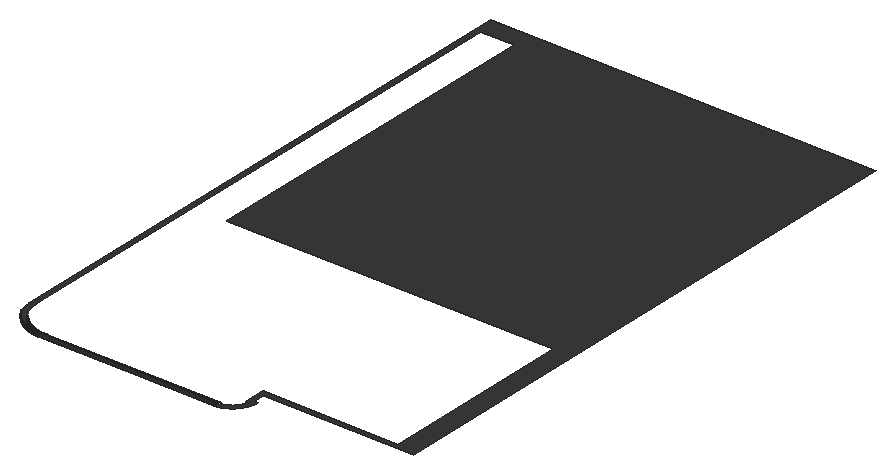
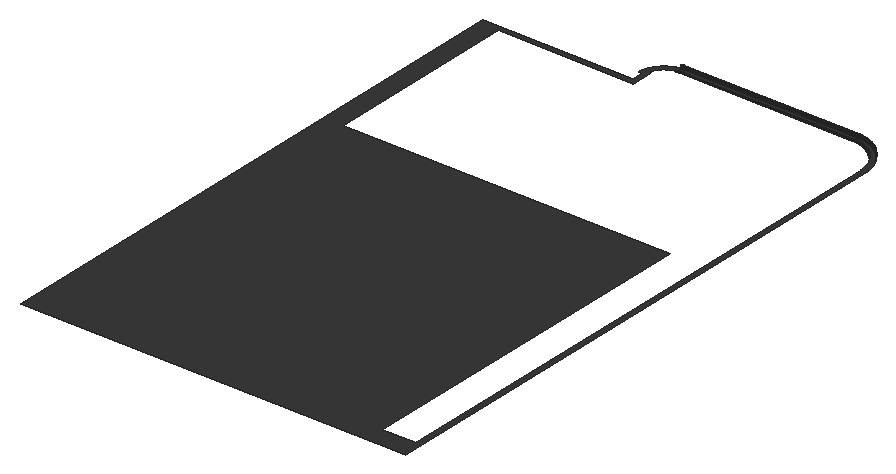
# SketchUp Ruby script. Lengths in inches.
U = 1.inch
M = Sketchup.active_model
def pt(a) = Geom::Point3d.new(a.map { |v| v * U })
def face(e, loops, mat)
  f = e.add_face(loops[0].map { |a| pt(a) })
  loops[1..].each { |l| e.add_face(l.map { |a| pt(a) }).erase! }
  f.material = f.back_material = mat if mat
  f
end
# faces: each face lists its corners as indices into pts; further lists are holes
def faces(e, pts, list, mat = nil) = list.each { |f| face(e, (f[0].is_a?(Array) ? f : [f]).map { |l| l.map { |i| pts[i] } }, mat) }
# xy, xz, yz: faces in a plane at the given z, y or x. An outline is a flat list of corners, or four numbers for a rectangle; further outlines are holes
def ring(l) = l.size == 4 ? [[l[0], l[1]], [l[2], l[1]], [l[2], l[3]], [l[0], l[3]]] : l.each_slice(2).to_a
def flat(e, list, mat, &to3) = list.each { |f| face(e, (f[0].is_a?(Array) ? f : [f]).map { |l| ring(l).map { |u, v| to3.(u, v) } }, mat) }
def xy(e, z, list, mat = nil) = flat(e, list, mat) { |x, y| [x, y, z] }
def xz(e, y, list, mat = nil) = flat(e, list, mat) { |x, z| [x, y, z] }
def yz(e, x, list, mat = nil) = flat(e, list, mat) { |y, z| [x, y, z] }
def lines(e, pts, list) = list.each { |a, b| e.add_line(pt(pts[a]), pt(pts[b])) }
# prism: a flat outline (further loops are holes) pulled along v
def prism(e, loops, v, mat = nil)
  f = face(e, loops, mat); d = Geom::Vector3d.new(v.map { |x| x * U })
  f.pushpull(f.normal.samedirection?(d) ? d.length : -d.length)
end
def box(e, o, s, mat = nil) = prism(e, [[o, [o[0] + s[0], o[1], o[2]], [o[0] + s[0], o[1] + s[1], o[2]], [o[0], o[1] + s[1], o[2]]]], [0, 0, s[2]], mat)
def at(x, y, z, deg = 0) = Geom::Transformation.translation(pt([x, y, z])) * Geom::Transformation.rotation(ORIGIN, Z_AXIS, deg.degrees)
def axes(o, x, y, z) = Geom::Transformation.new([*x, 0, *y, 0, *z, 0, *pt(o).to_a, 1])
def part(name) = M.definitions.add(name)
# library, detail: a bought-in or finely detailed component or shape, given as its bounding box
def library(name, o, s) = part(name).tap { |d| box(d.entities, o, s) }
def detail(e, o, s) = box(e.add_group.entities, o, s)
def put(e, d, t, mat = nil) = e.add_instance(d, t).tap { |i| i.material = mat if mat }
def group(e, t, mat = nil) = e.add_group.tap { |g| g.transformation = t; g.material = mat if mat }.entities
root = M.entities
M.materials.add("1496 AP 8293 CARBON COPY").color = [58, 58, 58]
xy(root,258,[[[43.57,64,43.14,64.01,42.7,64.03,41.84,64.07,41.41,64.1,40.55,64.18,39.69,64.28,39.26,64.34,38.84,64.41,38.41,64.48,37.99,64.55,37.5625,64.63,37.14,64.72,36.72,64.8125,36.3,64.91,35.875,65.02,35.46,65.125,35.04,65.24,34.63,65.36,34.21,65.48,33.8,65.62,33.39,65.75,32.98,65.89,32.58,66.04,32.17,66.19,31.37,66.51,30.97,66.68,30.58,66.85,30.18,67.03,29.79,67.21,29.4,67.4,29.02,67.6,28.63,67.8,28.25,68,27.5,68.42,26.76,68.86,26.39,69.09,26.03,69.32,25.67,69.5625,25.31,69.8,24.95,70.05,24.6,70.3,24.26,70.56,23.91,70.82,23.57,71.08,23.23,71.35,22.57,71.91,22.24,72.1875,21.92,72.48,21.6,72.77,21.28,73.0625,20.97,73.36,20.67,73.67,20.36,73.97,20.0625,74.28,19.77,74.6,19.48,74.92,19.1875,75.24,18.91,75.57,18.35,76.23,18.08,76.57,17.82,76.91,17.56,77.26,17.3,77.6,17.05,77.95,16.8,78.31,16.5625,78.67,16.32,79.03,16.09,79.39,15.86,79.76,15.42,80.5,15,81.25,14.8,81.63,14.6,82.02,14.4,82.4,14.21,82.79,14.03,83.18,13.85,83.58,13.68,83.97,13.51,84.37,13.19,85.17,13.04,85.58,12.89,85.98,12.75,86.39,12.62,86.8,12.48,87.21,12.36,87.63,12.24,88.04,12.125,88.46,12.02,88.875,11.91,89.3,11.8125,89.72,11.72,90.14,11.63,90.5625,11.55,90.99,11.48,91.41,11.41,91.84,11.34,92.26,11.28,92.69,11.18,93.55,11.1,94.41,11.07,94.84,11.03,95.7,11.01,96.14,11,96.57,11,567,326,567,326,94,203,94,203,85,206,85,206,84.73,205.99,84.45,205.98,84.18,205.97,83.9,205.96,83.625,205.94,83.35,205.91,83.08,205.88,82.8,205.82,82.26,205.78,81.99,205.74,81.71,205.7,81.44,205.6,80.9,205.54,80.63,205.48,80.37,205.42,80.1,205.28,79.56,205.14,79.04,205.06,78.77,204.97,78.51,204.89,78.25,204.8,77.99,204.7,77.73,204.61,77.47,204.51,77.22,204.4,76.96,204.07,76.21,203.83,75.71,203.71,75.47,203.58,75.22,203.46,74.98,203.32,74.74,203.1875,74.5,203.05,74.26,202.91,74.03,202.76,73.79,202.61,73.5625,202.46,73.33,202.31,73.11,202.15,72.88,201.83,72.44,201.32,71.78,201.15,71.57,200.79,71.15,200.61,70.95,200.42,70.75,200.23,70.54,200.04,70.35,199.85,70.15,199.65,69.96,199.46,69.77,199.25,69.58,199.05,69.39,198.85,69.21,198.43,68.85,198.22,68.68,197.56,68.17,197.12,67.85,196.89,67.69,196.67,67.54,196.4375,67.39,196.21,67.24,195.97,67.09,195.74,66.95,195.5,66.8125,195.26,66.68,195.02,66.54,194.78,66.42,194.53,66.29,194.29,66.17,193.79,65.93,193.04,65.6,192.78,65.49,192.53,65.39,192.27,65.3,192.01,65.2,191.75,65.11,191.49,65.03,191.23,64.94,190.96,64.86,190.44,64.72,189.9,64.58,189.63,64.52,189.37,64.46,189.1,64.4,188.56,64.3,188.29,64.26,188.01,64.22,187.74,64.18,187.2,64.12,186.92,64.09,186.65,64.06,186.375,64.04,186.1,64.03,185.82,64.02,185.55,64.01,185.27,64],[43.62,68,185.22,68,185.45,68.01,185.67,68.01,185.89,68.02,186.11,68.04,186.33,68.05,186.56,68.07,186.78,68.09,187.22,68.15,187.4375,68.18,187.66,68.21,187.88,68.25,188.1,68.28,188.32,68.33,188.53,68.37,188.97,68.47,189.18,68.52,189.4,68.58,189.61,68.64,189.83,68.7,190.04,68.76,190.46,68.9,190.67,68.98,190.88,69.05,191.51,69.29,191.91,69.47,192.12,69.5625,192.32,69.66,192.52,69.75,192.72,69.85,192.92,69.96,193.11,70.06,193.31,70.17,193.69,70.39,193.88,70.51,194.07,70.62,194.26,70.74,194.44,70.87,194.63,70.99,194.8125,71.12,194.99,71.25,195.35,71.51,195.52,71.65,195.7,71.79,196.04,72.07,196.21,72.22,196.54,72.52,196.86,72.82,197.18,73.14,197.48,73.46,197.78,73.79,197.93,73.96,198.21,74.3,198.35,74.48,198.49,74.65,198.75,75.01,198.88,75.1875,199.01,75.37,199.13,75.56,199.26,75.74,199.38,75.93,199.49,76.12,199.61,76.31,199.83,76.69,199.94,76.89,200.04,77.08,200.15,77.28,200.25,77.48,200.34,77.68,200.4375,77.88,200.53,78.09,200.71,78.49,200.95,79.12,201.02,79.33,201.1,79.54,201.24,79.96,201.3,80.17,201.36,80.39,201.42,80.6,201.48,80.82,201.52,81,199,81,199,98,310,98,310,257,43,257,43,551,15,551,15,96.62,15.02,95.86,15.04,95.48,15.0625,95.1,15.09,94.72,15.12,94.35,15.2,93.59,15.25,93.21,15.3,92.84,15.36,92.46,15.42,92.09,15.49,91.72,15.56,91.34,15.63,90.97,15.72,90.6,15.8,90.23,15.89,89.86,15.99,89.49,16.09,89.13,16.19,88.76,16.3,88.4,16.66,87.32,16.79,86.96,16.93,86.61,17.06,86.25,17.51,85.2,17.66,84.86,17.83,84.52,17.99,84.17,18.16,83.83,18.34,83.5,18.51,83.16,19.08,82.17,19.27,81.85,19.47,81.53,20.1,80.57,20.54,79.95,20.76,79.65,20.99,79.35,21.23,79.05,21.46,78.75,21.7,78.46,22.2,77.88,22.45,77.6,22.7,77.31,22.96,77.04,23.23,76.76,23.49,76.49,23.76,76.23,24.04,75.96,24.31,75.7,24.6,75.45,24.88,75.2,25.46,74.7,25.75,74.46,26.05,74.23,26.35,73.99,26.65,73.76,26.95,73.54,27.57,73.1,28.53,72.47,28.85,72.27,29.17,72.08,30.16,71.51,30.5,71.34,30.83,71.16,31.17,70.99,31.52,70.83,31.86,70.66,32.2,70.51,33.25,70.06,33.61,69.93,33.96,69.79,34.32,69.66,35.4,69.3,35.76,69.19,36.13,69.09,36.49,68.99,36.86,68.89,37.23,68.8,37.6,68.72,37.97,68.63,38.34,68.56,38.72,68.49,39.09,68.42,39.46,68.36,39.84,68.3,40.21,68.25,40.59,68.2,41.35,68.12,41.72,68.09,42.1,68.0625,42.48,68.04,42.86,68.02]]],"1496 AP 8293 CARBON COPY")
xz(root,64,[[43.57,258,44,261],[44,258,185,261],[185,258,185.27,261]],"1496 AP 8293 CARBON COPY")
xz(root,68,[[43.62,258,44,258.5],[44,258,184.99,258.5],[184.99,258,185.22,258.5]])
xz(root,68.01,[[185.45,258,185.67,258.5]])
xz(root,69,[[43.63,258,44,258.5],[44,258,184.98,258.5],[184.98,258,185.21,258.5]])
xz(root,69.01,[[185.42,258,185.63,258.5]])
p = [[42.27,64.05,261],[41.84,64.07,261],[41.84,64.07,258],[42.27,64.05,258],[42.7,64.03,261],[42.7,64.03,258],
  [43.14,64.01,261],[43.14,64.01,258],[43.57,64,261],[43.57,64,258],[185.55,64.01,261],[185.27,64,261],
  [185.27,64,258],[185.55,64.01,258],[185.82,64.02,261],[185.82,64.02,258],[186.1,64.03,261],[186.1,64.03,258],
  [186.375,64.04,261],[186.375,64.04,258],[186.65,64.06,261],[186.65,64.06,258],[40.98,64.14,261],[40.55,64.18,261],
  [40.55,64.18,258],[40.98,64.14,258],[41.41,64.1,261],[41.41,64.1,258],[186.92,64.09,261],[186.92,64.09,258],
  [187.2,64.12,261],[187.2,64.12,258],[187.47,64.15,261],[187.47,64.15,258],[187.74,64.18,261],[187.74,64.18,258],
  [40.12,64.23,261],[39.69,64.28,261],[39.69,64.28,258],[40.12,64.23,258],[39.26,64.34,261],[38.84,64.41,261],
  [38.84,64.41,258],[39.26,64.34,258],[38.41,64.48,261],[38.41,64.48,258],[37.99,64.55,261],[37.99,64.55,258],
  [37.5625,64.63,261],[37.14,64.72,261],[37.14,64.72,258],[37.5625,64.63,258],[36.72,64.8125,261],[36.72,64.8125,258],
  [36.3,64.91,261],[36.3,64.91,258],[35.875,65.02,261],[35.875,65.02,258],[35.46,65.125,261],[35.46,65.125,258],
  [35.04,65.24,261],[35.04,65.24,258],[34.63,65.36,261],[34.63,65.36,258],[34.21,65.48,261],[34.21,65.48,258],
  [33.8,65.62,261],[33.8,65.62,258],[33.39,65.75,261],[33.39,65.75,258],[32.98,65.89,261],[32.98,65.89,258],
  [32.58,66.04,261],[32.58,66.04,258],[32.17,66.19,261],[32.17,66.19,258],[31.77,66.35,261],[31.77,66.35,258],
  [31.37,66.51,261],[31.37,66.51,258],[30.97,66.68,261],[30.97,66.68,258],[30.58,66.85,261],[30.58,66.85,258],
  [30.18,67.03,261],[30.18,67.03,258],[29.79,67.21,261],[29.79,67.21,258],[29.4,67.4,261],[29.4,67.4,258],
  [29.02,67.6,261],[29.02,67.6,258],[28.63,67.8,261],[28.63,67.8,258],[28.25,68,261],[28.25,68,258],
  [27.875,68.21,261],[27.875,68.21,258],[42.48,68.04,258],[42.1,68.0625,258],[42.1,68.0625,258.5],[42.48,68.04,258.5],
  [42.86,68.02,258],[42.86,68.02,258.5],[43.24,68.01,258],[43.24,68.01,258.5],[43.62,68,258],[43.62,68,258.5],
  [185.45,68.01,258],[185.22,68,258],[185.22,68,258.5],[185.45,68.01,258.5],[185.89,68.02,258],[185.67,68.01,258],
  [185.67,68.01,258.5],[185.89,68.02,258.5],[186.11,68.04,258],[186.11,68.04,258.5],[186.33,68.05,258],[186.33,68.05,258.5],
  [41.35,68.12,258],[40.97,68.16,258],[40.97,68.16,258.5],[41.35,68.12,258.5],[41.72,68.09,258],[41.72,68.09,258.5],
  [186.56,68.07,258],[186.56,68.07,258.5],[186.78,68.09,258],[186.78,68.09,258.5],[187,68.12,258],[187,68.12,258.5],
  [187.22,68.15,258],[187.22,68.15,258.5],[187.4375,68.18,258],[187.4375,68.18,258.5],[27.5,68.42,261],[27.5,68.42,258],
  [40.21,68.25,258],[39.84,68.3,258],[39.84,68.3,258.5],[40.21,68.25,258.5],[40.59,68.2,258],[40.59,68.2,258.5],
  [187.66,68.21,258],[187.66,68.21,258.5],[39.46,68.36,258],[39.46,68.36,258.5],[27.13,68.64,261],[27.13,68.64,258],
  [39.09,68.42,258],[38.72,68.49,258],[38.72,68.49,258.5],[39.09,68.42,258.5],[38.34,68.56,258],[38.34,68.56,258.5],
  [26.76,68.86,261],[26.76,68.86,258],[37.97,68.63,258],[37.6,68.72,258],[37.6,68.72,258.5],[37.97,68.63,258.5],
  [37.23,68.8,258],[37.23,68.8,258.5],[36.86,68.89,258],[36.86,68.89,258.5],[26.39,69.09,261],[26.39,69.09,258],
  [36.49,68.99,258],[36.49,68.99,258.5],[36.13,69.09,258],[36.13,69.09,258.5],[42.17,69.06,258],[42.53,69.04,258],
  [42.53,69.04,258.5],[42.17,69.06,258.5],[42.9,69.02,258],[42.9,69.02,258.5],[43.27,69.01,258],[43.27,69.01,258.5],
  [43.63,69,258],[43.63,69,258.5],[185.21,69,258],[185.42,69.01,258],[185.42,69.01,258.5],[185.21,69,258.5],
  [185.63,69.01,258],[185.84,69.02,258],[185.84,69.02,258.5],[185.63,69.01,258.5],[186.05,69.03,258],[186.05,69.03,258.5],
  [186.26,69.05,258],[186.26,69.05,258.5],[186.46,69.07,258],[186.46,69.07,258.5],[26.03,69.32,261],[26.03,69.32,258],
  [35.76,69.19,258],[35.76,69.19,258.5],[41.07,69.15,258],[41.4375,69.12,258],[41.4375,69.12,258.5],[41.07,69.15,258.5],
  [41.8,69.09,258],[41.8,69.09,258.5],[186.67,69.09,258],[186.67,69.09,258.5],[186.88,69.11,258],[186.88,69.11,258.5],
  [187.09,69.14,258],[187.09,69.14,258.5],[187.3,69.17,258],[187.3,69.17,258.5],[35.4,69.3,258],[35.4,69.3,258.5],
  [39.98,69.29,258],[40.35,69.24,258],[40.35,69.24,258.5],[39.98,69.29,258.5],[40.71,69.19,258],[40.71,69.19,258.5],
  [187.5,69.2,258],[187.5,69.2,258.5],[187.71,69.23,258],[187.71,69.23,258.5],[25.67,69.5625,261],[25.67,69.5625,258],
  [35.04,69.42,258],[35.04,69.42,258.5],[39.26,69.4,258],[39.62,69.34,258],[39.62,69.34,258.5],[39.26,69.4,258.5],
  [34.68,69.54,258],[34.68,69.54,258.5],[38.9,69.47,258],[38.9,69.47,258.5],[34.32,69.66,258],[34.32,69.66,258.5],
  [38.18,69.61,258],[38.54,69.54,258],[38.54,69.54,258.5],[38.18,69.61,258.5],[25.31,69.8,261],[25.31,69.8,258],
  [37.82,69.69,258],[37.82,69.69,258.5],[33.96,69.79,258],[33.96,69.79,258.5],[37.46,69.77,258],[37.46,69.77,258.5],
  [24.95,70.05,261],[24.95,70.05,258],[33.61,69.93,258],[33.61,69.93,258.5],[37.11,69.86,258],[37.11,69.86,258.5],
  [33.25,70.06,258],[33.25,70.06,258.5],[36.75,69.95,258],[36.75,69.95,258.5],[36.4,70.05,258],[36.4,70.05,258.5],
  [24.6,70.3,261],[24.6,70.3,258],[32.9,70.21,258],[32.9,70.21,258.5],[36.05,70.15,258],[36.05,70.15,258.5],
  [32.55,70.36,258],[32.55,70.36,258.5],[35.7,70.26,258],[35.7,70.26,258.5],[24.26,70.56,261],[24.26,70.56,258],
  [35.35,70.37,258],[35.35,70.37,258.5],[32.2,70.51,258],[32.2,70.51,258.5],[35,70.49,258],[35,70.49,258.5],
  [31.86,70.66,258],[31.86,70.66,258.5],[34.65,70.61,258],[34.65,70.61,258.5],[23.91,70.82,261],[23.91,70.82,258],
  [34.31,70.73,258],[34.31,70.73,258.5],[31.52,70.83,258],[31.52,70.83,258.5],[33.97,70.86,258],[33.97,70.86,258.5],
  [23.57,71.08,261],[23.57,71.08,258],[31.17,70.99,258],[31.17,70.99,258.5],[33.625,70.99,258],[33.625,70.99,258.5],
  [30.83,71.16,258],[30.83,71.16,258.5],[33.28,71.13,258],[33.28,71.13,258.5],[23.23,71.35,261],[23.23,71.35,258],
  [32.95,71.27,258],[32.95,71.27,258.5],[30.5,71.34,258],[30.5,71.34,258.5],[30.16,71.51,258],[30.16,71.51,258.5],
  [32.61,71.42,258],[32.61,71.42,258.5],[22.9,71.63,261],[22.9,71.63,258],[32.28,71.57,258],[32.28,71.57,258.5],
  [29.83,71.7,258],[29.83,71.7,258.5],[22.57,71.91,261],[22.57,71.91,258],[31.95,71.73,258],[31.95,71.73,258.5],
  [29.5,71.89,258],[29.5,71.89,258.5],[31.62,71.89,258],[31.62,71.89,258.5],[22.24,72.1875,261],[22.24,72.1875,258],
  [29.17,72.08,258],[29.17,72.08,258.5],[31.29,72.05,258],[31.29,72.05,258.5],[28.85,72.27,258],[28.85,72.27,258.5],
  [30.96,72.22,258],[30.96,72.22,258.5],[21.92,72.48,261],[21.92,72.48,258],[30.64,72.39,258],[30.64,72.39,258.5],
  [28.53,72.47,258],[28.53,72.47,258.5],[30.32,72.57,258],[30.32,72.57,258.5],[21.6,72.77,261],[21.6,72.77,258],
  [28.21,72.68,258],[28.21,72.68,258.5],[30,72.75,258],[30,72.75,258.5],[27.89,72.89,258],[27.89,72.89,258.5],
  [21.28,73.0625,261],[21.28,73.0625,258],[29.68,72.9375,258],[29.68,72.9375,258.5],[27.57,73.1,258],[27.57,73.1,258.5],
  [29.37,73.125,258],[29.37,73.125,258.5],[20.97,73.36,261],[20.97,73.36,258],[27.26,73.32,258],[27.26,73.32,258.5],
  [29.06,73.32,258],[29.06,73.32,258.5],[26.95,73.54,258],[26.95,73.54,258.5],[28.75,73.52,258],[28.75,73.52,258.5],
  [20.67,73.67,261],[20.67,73.67,258],[26.65,73.76,258],[26.65,73.76,258.5],[28.44,73.72,258],[28.44,73.72,258.5],
  [20.36,73.97,261],[20.36,73.97,258],[28.14,73.92,258],[28.14,73.92,258.5],[26.35,73.99,258],[26.35,73.99,258.5],
  [27.84,74.13,258],[27.84,74.13,258.5],[20.0625,74.28,261],[20.0625,74.28,258],[26.05,74.23,258],[26.05,74.23,258.5],
  [27.54,74.35,258],[27.54,74.35,258.5],[25.75,74.46,258],[25.75,74.46,258.5],[19.77,74.6,261],[19.77,74.6,258],
  [27.25,74.56,258],[27.25,74.56,258.5],[25.46,74.7,258],[25.46,74.7,258.5],[19.48,74.92,261],[19.48,74.92,258],
  [26.95,74.79,258],[26.95,74.79,258.5],[25.17,74.95,258],[25.17,74.95,258.5],[26.67,75.01,258],[26.67,75.01,258.5],
  [19.1875,75.24,261],[19.1875,75.24,258],[24.88,75.2,258],[24.88,75.2,258.5],[26.38,75.24,258],[26.38,75.24,258.5],
  [18.91,75.57,261],[18.91,75.57,258],[24.6,75.45,258],[24.6,75.45,258.5],[26.1,75.47,258],[26.1,75.47,258.5],
  [24.31,75.7,258],[24.31,75.7,258.5],[25.82,75.71,258],[25.82,75.71,258.5],[18.63,75.9,261],[18.63,75.9,258],
  [24.04,75.96,258],[24.04,75.96,258.5],[25.54,75.95,258],[25.54,75.95,258.5],[18.35,76.23,261],[18.35,76.23,258],
  [25.26,76.19,258],[25.26,76.19,258.5],[23.76,76.23,258],[23.76,76.23,258.5],[18.08,76.57,261],[18.08,76.57,258],
  [23.49,76.49,258],[23.49,76.49,258.5],[24.99,76.4375,258],[24.99,76.4375,258.5],[24.73,76.69,258],[24.73,76.69,258.5],
  [23.23,76.76,258],[23.23,76.76,258.5],[17.82,76.91,261],[17.82,76.91,258],[24.46,76.94,258],[24.46,76.94,258.5],
  [22.96,77.04,258],[22.96,77.04,258.5],[17.56,77.26,261],[17.56,77.26,258],[24.2,77.2,258],[24.2,77.2,258.5],
  [22.7,77.31,258],[22.7,77.31,258.5],[23.94,77.46,258],[23.94,77.46,258.5],[17.3,77.6,261],[17.3,77.6,258],
  [22.45,77.6,258],[22.45,77.6,258.5],[23.69,77.73,258],[23.69,77.73,258.5],[17.05,77.95,261],[17.05,77.95,258],
  [22.2,77.88,258],[22.2,77.88,258.5],[23.4375,77.99,258],[23.4375,77.99,258.5],[21.95,78.17,258],[21.95,78.17,258.5],
  [16.8,78.31,261],[16.8,78.31,258],[23.19,78.26,258],[23.19,78.26,258.5],[21.7,78.46,258],[21.7,78.46,258.5],
  [16.5625,78.67,261],[16.5625,78.67,258],[22.95,78.54,258],[22.95,78.54,258.5],[21.46,78.75,258],[21.46,78.75,258.5],
  [22.71,78.82,258],[22.71,78.82,258.5],[16.32,79.03,261],[16.32,79.03,258],[21.23,79.05,258],[21.23,79.05,258.5],
  [22.47,79.1,258],[22.47,79.1,258.5],[16.09,79.39,261],[16.09,79.39,258],[20.99,79.35,258],[20.99,79.35,258.5],
  [22.24,79.38,258],[22.24,79.38,258.5],[20.76,79.65,258],[20.76,79.65,258.5],[15.86,79.76,261],[15.86,79.76,258],
  [22.01,79.67,258],[22.01,79.67,258.5],[20.54,79.95,258],[20.54,79.95,258.5],[21.79,79.95,258],[21.79,79.95,258.5],
  [15.64,80.13,261],[15.64,80.13,258],[20.32,80.26,258],[20.32,80.26,258.5],[21.56,80.25,258],[21.56,80.25,258.5],
  [15.42,80.5,261],[15.42,80.5,258],[21.35,80.54,258],[21.35,80.54,258.5]]
faces(root,p,[[0,1,2,3],[4,0,3,5],[6,4,5,7],[8,6,7,9],[10,11,12,13],[14,10,13,15],[16,14,15,17],[18,16,17,19],
  [20,18,19,21],[22,23,24,25],[26,22,25,27],[1,26,27,2],[28,20,21,29],[30,28,29,31],[32,30,31,33],[34,32,33,35],
  [36,37,38,39],[23,36,39,24],[40,41,42,43],[37,40,43,38],[41,44,45,42],[44,46,47,45],[48,49,50,51],[46,48,51,47],
  [49,52,53,50],[52,54,55,53],[54,56,57,55],[56,58,59,57],[58,60,61,59],[60,62,63,61],[62,64,65,63],[64,66,67,65],
  [66,68,69,67],[68,70,71,69],[70,72,73,71],[72,74,75,73],[74,76,77,75],[76,78,79,77],[78,80,81,79],[80,82,83,81],
  [82,84,85,83],[84,86,87,85],[86,88,89,87],[88,90,91,89],[90,92,93,91],[92,94,95,93],[94,96,97,95],[96,136,137,97],
  [136,148,149,137],[148,156,157,149],[156,166,167,157],[166,196,197,167],[196,226,227,197],[226,244,245,227],[244,252,253,245],[252,264,265,253],
  [264,274,275,265],[274,286,287,275],[286,294,295,287],[294,304,305,295],[304,314,315,305],[314,320,321,315],[320,328,329,321],[328,338,339,329],
  [338,346,347,339],[346,354,355,347],[354,362,363,355],[362,372,373,363],[372,378,379,373],[378,386,387,379],[386,394,395,387],[394,400,401,395],
  [400,408,409,401],[408,414,415,409],[414,424,425,415],[424,430,431,425],[430,436,437,431],[436,446,447,437],[446,452,453,447],[452,460,461,453],
  [460,466,467,461],[466,474,475,467],[474,480,481,475],[480,488,489,481],[488,494,495,489],[494,502,503,495],[502,510,511,503],[510,516,517,511]],"1496 AP 8293 CARBON COPY")
faces(root,p,[[98,99,100,101],[102,98,101,103],[104,102,103,105],[106,104,105,107],[108,109,110,111],[112,113,114,115],[116,112,115,117],[118,116,117,119],
  [120,121,122,123],[124,120,123,125],[99,124,125,100],[126,118,119,127],[128,126,127,129],[130,128,129,131],[132,130,131,133],[134,132,133,135],
  [138,139,140,141],[142,138,141,143],[121,142,143,122],[144,134,135,145],[139,146,147,140],[150,151,152,153],[146,150,153,147],[151,154,155,152],
  [158,159,160,161],[154,158,161,155],[159,162,163,160],[162,164,165,163],[164,168,169,165],[168,170,171,169],[172,173,174,175],[173,176,177,174],
  [176,178,179,177],[178,180,181,179],[182,183,184,185],[186,187,188,189],[187,190,191,188],[190,192,193,191],[192,194,195,193],[170,198,199,171],
  [200,201,202,203],[201,204,205,202],[204,172,175,205],[194,206,207,195],[206,208,209,207],[208,210,211,209],[210,212,213,211],[198,214,215,199],
  [216,217,218,219],[217,220,221,218],[220,200,203,221],[212,222,223,213],[222,224,225,223],[214,228,229,215],[230,231,232,233],[231,216,219,232],
  [228,234,235,229],[236,230,233,237],[234,238,239,235],[240,241,242,243],[241,236,237,242],[246,240,243,247],[238,248,249,239],[250,246,247,251],
  [248,254,255,249],[256,250,251,257],[254,258,259,255],[260,256,257,261],[262,260,261,263],[258,266,267,259],[268,262,263,269],[266,270,271,267],
  [272,268,269,273],[276,272,273,277],[270,278,279,271],[280,276,277,281],[278,282,283,279],[284,280,281,285],[288,284,285,289],[282,290,291,283],
  [292,288,289,293],[290,296,297,291],[298,292,293,299],[296,300,301,297],[302,298,299,303],[306,302,303,307],[300,308,309,301],[308,310,311,309],
  [312,306,307,313],[316,312,313,317],[310,318,319,311],[322,316,317,323],[318,324,325,319],[326,322,323,327],[324,330,331,325],[332,326,327,333],
  [330,334,335,331],[336,332,333,337],[340,336,337,341],[334,342,343,335],[344,340,341,345],[342,348,349,343],[350,344,345,351],[348,352,353,349],
  [356,350,351,357],[352,358,359,353],[360,356,357,361],[358,364,365,359],[366,360,361,367],[364,368,369,365],[370,366,367,371],[368,374,375,369],
  [376,370,371,377],[380,376,377,381],[374,382,383,375],[384,380,381,385],[382,388,389,383],[390,384,385,391],[388,392,393,389],[396,390,391,397],
  [392,398,399,393],[402,396,397,403],[398,404,405,399],[406,402,403,407],[404,410,411,405],[412,406,407,413],[410,416,417,411],[418,412,413,419],
  [416,420,421,417],[422,418,419,423],[420,426,427,421],[428,422,423,429],[432,428,429,433],[426,434,435,427],[434,438,439,435],[440,432,433,441],
  [442,440,441,443],[438,444,445,439],[448,442,443,449],[444,450,451,445],[454,448,449,455],[450,456,457,451],[458,454,455,459],[456,462,463,457],
  [464,458,459,465],[462,468,469,463],[470,464,465,471],[468,472,473,469],[476,470,471,477],[472,478,479,473],[482,476,477,483],[478,484,485,479],
  [486,482,483,487],[484,490,491,485],[492,486,487,493],[490,496,497,491],[498,492,493,499],[496,500,501,497],[504,498,499,505],[500,506,507,501],
  [508,504,505,509],[506,512,513,507],[514,508,509,515],[518,514,515,519]])
